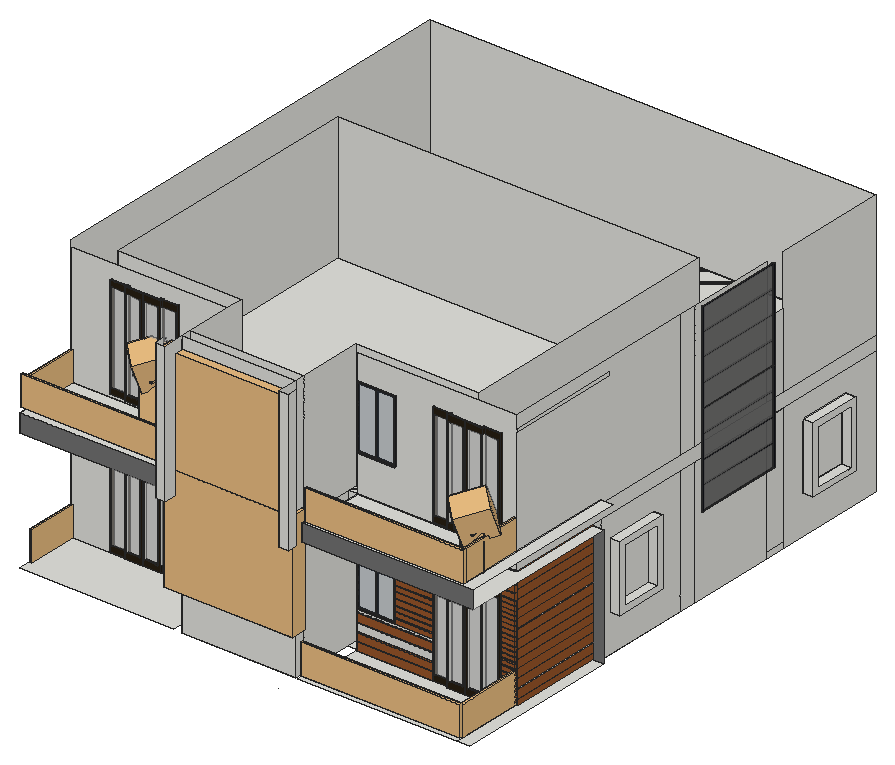
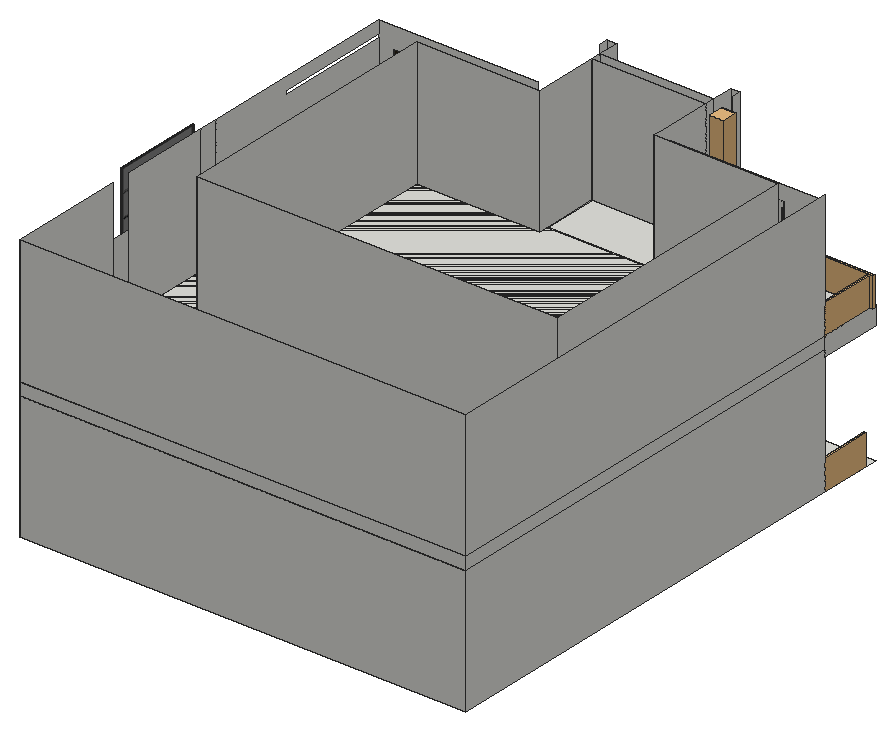
# SketchUp Ruby script. Lengths in inches.
U = 1.inch
M = Sketchup.active_model
def pt(a) = Geom::Point3d.new(a.map { |v| v * U })
def face(e, loops, mat)
  f = e.add_face(loops[0].map { |a| pt(a) })
  loops[1..].each { |l| e.add_face(l.map { |a| pt(a) }).erase! }
  f.material = f.back_material = mat if mat
  f
end
# faces: each face lists its corners as indices into pts; further lists are holes
def faces(e, pts, list, mat = nil) = list.each { |f| face(e, (f[0].is_a?(Array) ? f : [f]).map { |l| l.map { |i| pts[i] } }, mat) }
# xy, xz, yz: faces in a plane at the given z, y or x. An outline is a flat list of corners, or four numbers for a rectangle; further outlines are holes
def ring(l) = l.size == 4 ? [[l[0], l[1]], [l[2], l[1]], [l[2], l[3]], [l[0], l[3]]] : l.each_slice(2).to_a
def flat(e, list, mat, &to3) = list.each { |f| face(e, (f[0].is_a?(Array) ? f : [f]).map { |l| ring(l).map { |u, v| to3.(u, v) } }, mat) }
def xy(e, z, list, mat = nil) = flat(e, list, mat) { |x, y| [x, y, z] }
def xz(e, y, list, mat = nil) = flat(e, list, mat) { |x, z| [x, y, z] }
def yz(e, x, list, mat = nil) = flat(e, list, mat) { |y, z| [x, y, z] }
def lines(e, pts, list) = list.each { |a, b| e.add_line(pt(pts[a]), pt(pts[b])) }
# prism: a flat outline (further loops are holes) pulled along v
def prism(e, loops, v, mat = nil)
  f = face(e, loops, mat); d = Geom::Vector3d.new(v.map { |x| x * U })
  f.pushpull(f.normal.samedirection?(d) ? d.length : -d.length)
end
def box(e, o, s, mat = nil) = prism(e, [[o, [o[0] + s[0], o[1], o[2]], [o[0] + s[0], o[1] + s[1], o[2]], [o[0], o[1] + s[1], o[2]]]], [0, 0, s[2]], mat)
def at(x, y, z, deg = 0) = Geom::Transformation.translation(pt([x, y, z])) * Geom::Transformation.rotation(ORIGIN, Z_AXIS, deg.degrees)
def axes(o, x, y, z) = Geom::Transformation.new([*x, 0, *y, 0, *z, 0, *pt(o).to_a, 1])
def part(name) = M.definitions.add(name)
# library, detail: a bought-in or finely detailed component or shape, given as its bounding box
def library(name, o, s) = part(name).tap { |d| box(d.entities, o, s) }
def detail(e, o, s) = box(e.add_group.entities, o, s)
def put(e, d, t, mat = nil) = e.add_instance(d, t).tap { |i| i.material = mat if mat }
def group(e, t, mat = nil) = e.add_group.tap { |g| g.transformation = t; g.material = mat if mat }.entities
root = M.entities
M.materials.add("Material__1").color = [51, 42, 44]
M.materials.add("Material__2").color = [97, 132, 37]
M.materials.add("[0136_Charcoal]").color = [35, 35, 35]
M.materials.add("[Color M05]").color = [114, 114, 114]
M.materials.add("[Translucent Glass Gray]2").color = [201, 201, 201]
M.materials["[Translucent Glass Gray]2"].alpha = 0.5
M.materials.add("[Translucent_Glass_Blue]").color = [68, 104, 165]
M.materials["[Translucent_Glass_Blue]"].alpha = 0.07
M.materials.add("[Translucent_Glass_Green_Dark]").color = [33, 68, 103]
M.materials["[Translucent_Glass_Green_Dark]"].alpha = 0.08
M.materials.add("[Wood Cherry Original]").color = [152, 86, 42]
M.materials.add("oak swatch").color = [40, 31, 19]
M.materials.add("{045efeae-c101-a24d-bd9b-6f5600100adb}").color = [102, 102, 102]
M.materials["{045efeae-c101-a24d-bd9b-6f5600100adb}"].alpha = 0.7
M.materials.add("{16756a1b-d383-d94f-ad82-104813d2624f}").color = [19, 21, 27]
c1 = part("Group\#7")
box(c1.entities,[0,0,0],[1.77,4.72,80.31],"oak swatch")
c2 = part("Exterior Sliding Doors")
xy(c2.entities,0,[[1.77,33.07,3.54,70.87],[1.77,70.87,3.54,108.66]])
xy(c2.entities,0,[[0,0,1.77,33.07],[0,108.66,1.77,141.73]],"oak swatch")
xy(c2.entities,4.72,[[0,4.72,1.77,33.07],[1.77,37.8,3.54,66.14],[1.77,75.88,3.54,103.9375],[0,108.66,1.77,137.01]],"oak swatch")
xy(c2.entities,75.59,[[1.77,37.8,3.54,66.14],[1.77,75.88,3.54,103.9375]])
xy(c2.entities,75.59,[[0,4.72,1.77,33.07],[0,108.66,1.77,137.01]],"oak swatch")
xy(c2.entities,80.31,[[0,0,1.77,33.07],[1.77,33.07,3.54,70.87],[1.77,70.87,3.54,108.66],[0,108.66,1.77,141.73]],"oak swatch")
xz(c2.entities,0,[[0,0,1.77,80.31]],"oak swatch")
xz(c2.entities,4.72,[[0,4.72,1.77,75.59]],"oak swatch")
xz(c2.entities,33.07,[[0,0,1.77,4.72],[1.77,0,3.54,80.31],[0,75.59,1.77,80.31]],"oak swatch")
xz(c2.entities,37.8,[[1.77,4.72,3.54,75.59]])
xz(c2.entities,66.14,[[1.77,4.72,3.54,75.59]],"oak swatch")
xz(c2.entities,70.87,[[1.77,0,3.54,80.31]])
xz(c2.entities,75.88,[[1.77,4.72,3.54,75.59]])
xz(c2.entities,103.9375,[[1.77,4.72,3.54,75.59]],"oak swatch")
xz(c2.entities,108.66,[[1.77,4.72,3.54,75.59]])
xz(c2.entities,108.66,[[0,0,3.54,4.72],[0,75.59,3.54,80.31]],"oak swatch")
xz(c2.entities,137.01,[[0,4.72,1.77,75.59]],"oak swatch")
xz(c2.entities,141.73,[[0,0,1.77,80.31]],"oak swatch")
yz(c2.entities,0,[[0,0,33.07,0,33.07,4.72,4.72,4.72,4.72,75.59,33.07,75.59,33.07,80.31,0,80.31],[108.66,0,141.73,0,141.73,80.31,108.66,80.31,108.66,75.59,137.01,75.59,137.01,4.72,108.66,4.72]],"oak swatch")
yz(c2.entities,1.77,[[4.72,4.72,33.07,75.59],[37.8,4.72,66.14,75.59],[75.88,4.72,103.9375,75.59],[108.66,4.72,137.01,75.59]],"[Translucent Glass Gray]2")
yz(c2.entities,1.77,[[0,0,33.07,0,33.07,4.72,4.72,4.72,4.72,75.59,33.07,75.59,33.07,80.31,0,80.31],[[33.07,0,70.87,80.31],[37.8,4.72,66.14,75.59]],[[70.87,0,141.73,80.31],[108.66,4.72,137.01,75.59],[75.88,4.72,103.9375,75.59]]],"oak swatch")
yz(c2.entities,3.54,[[[33.07,0,70.87,80.31],[37.8,4.72,66.14,75.59]],[[70.87,0,108.66,80.31],[75.88,4.72,103.9375,75.59]]],"oak swatch")
put(c2.entities,c1,at(0,33.07,0))
put(c2.entities,c1,at(0,103.9375,0))
c3 = part("Group\#9")
box(c3.entities,[0,-1.5625,0],[72.51,1.5625,7.17])
c4 = library("Glass Railings(black Handrails)",[-57.04,-132.55,0],[169.29,2.52,28.17])
c5 = part("Group\#11")
box(c5.entities,[0,0,0],[14,3.63,1.625])
c6 = part("Group\#8")
box(c6.entities,[61.69,-1.625,-2],[88.94,1.625,7.49])
c7 = part("Group\#10")
box(c7.entities,[0,0,0],[36.2,4.62,1.5625])
c8 = part("Two-panel window \#1")
xy(c8.entities,-18,[[0,-31,2,35]],"[0136_Charcoal]")
xy(c8.entities,-16,[[0,-29,0.9375,33],[0.9375,-29,1.125,33],[1.125,-29,2,1],[1.125,3,2,33]],"[0136_Charcoal]")
xy(c8.entities,76,[[0,-29,0.9375,33],[0.9375,-29,1.125,33],[1.125,-29,2,1],[1.125,3,2,33]],"[0136_Charcoal]")
xy(c8.entities,78,[[0,-31,2,35]],"[0136_Charcoal]")
xz(c8.entities,-31,[[0,-18,2,78]],"[0136_Charcoal]")
xz(c8.entities,-29,[[0,-16,0.9375,76],[0.9375,-16,1.125,76],[1.125,-16,2,76]],"[0136_Charcoal]")
xz(c8.entities,1,[[1.125,-16,2,76]],"[0136_Charcoal]")
xz(c8.entities,3,[[1.125,-16,2,76]],"[0136_Charcoal]")
xz(c8.entities,33,[[0,-16,0.9375,76],[0.9375,-16,1.125,76],[1.125,-16,2,76]],"[0136_Charcoal]")
xz(c8.entities,35,[[0,-18,2,78]],"[0136_Charcoal]")
yz(c8.entities,0,[[[-31,-18,35,78],[-29,-16,33,76]]],"[0136_Charcoal]")
yz(c8.entities,0.9375,[[-29,-16,33,76]],"[Translucent_Glass_Blue]")
yz(c8.entities,1.125,[[1,-16,3,76]],"[0136_Charcoal]")
yz(c8.entities,1.125,[[-29,-16,1,76],[3,-16,33,76]],"[Translucent_Glass_Green_Dark]")
yz(c8.entities,2,[[[-31,-18,35,78],[-29,-16,1,76],[3,-16,33,76]]],"[0136_Charcoal]")
c9 = part("Two-panel window")
put(c9.entities,c8,axes([-31.84,50.72,0],[1,0,0],[0,1.1,0],[0,0,1]))
c10 = part("normal window")
put(c10.entities,c9,axes([114.26,44.3125,18],[0,1,0],[-0.90909,0,0],[0,0,1]))
c11 = part("Group\#20")
xy(c11.entities,0,[[[0,0,50.8125,62.9375],[5.49,5.49,45.32,57.45]],[5.49,5.49,45.32,57.45]])
xy(c11.entities,9.5625,[[[0,0,50.8125,62.9375],[5.49,5.49,45.32,57.45]]])
xz(c11.entities,0,[[0,0,50.8125,9.5625]])
xz(c11.entities,5.49,[[5.49,0,45.32,9.5625]])
xz(c11.entities,57.45,[[5.49,0,45.32,9.5625]])
xz(c11.entities,62.9375,[[0,0,50.8125,9.5625]])
yz(c11.entities,0,[[0,0,62.9375,9.5625]])
yz(c11.entities,5.49,[[5.49,0,57.45,9.5625]])
yz(c11.entities,45.32,[[5.49,0,57.45,9.5625]])
yz(c11.entities,50.8125,[[0,0,62.9375,9.5625]])
c12 = library("Facade Louver",[-2.17,-1,-2.17],[122.45,14.39,102.76])
c13 = part("Furniture_0DcpanrIvuI8n_9Ae92L5A")
g1 = group(c13.entities,at(0,0,0))
box(g1,[-19.29,-0.2,0.39],[38.58,0.4,83.86],"{045efeae-c101-a24d-bd9b-6f5600100adb}")
g2 = group(c13.entities,at(0,0,0))
box(g2,[-19.68,-0.59,63.39],[39.36,1.18,0.39],"{16756a1b-d383-d94f-ad82-104813d2624f}")
box(g2,[-19.68,-0.59,42.52],[39.36,1.18,0.39],"{16756a1b-d383-d94f-ad82-104813d2624f}")
box(g2,[-19.68,-0.59,21.26],[39.36,1.18,0.39],"{16756a1b-d383-d94f-ad82-104813d2624f}")
xy(g2,0,[[-19.68,-0.59,19.68,0.59]],"{16756a1b-d383-d94f-ad82-104813d2624f}")
xy(g2,0.39,[[-19.68,-0.59,-19.29,0.59],[-19.68,-0.59,19.68,0.59],[19.29,-0.59,19.68,0.59]],"{16756a1b-d383-d94f-ad82-104813d2624f}")
xy(g2,84.25,[[-19.68,-0.59,19.68,0.59]],"{16756a1b-d383-d94f-ad82-104813d2624f}")
xy(g2,84.65,[[-19.68,-0.59,-19.29,0.59],[-19.68,-0.59,19.68,0.59],[19.29,-0.59,19.68,0.59]],"{16756a1b-d383-d94f-ad82-104813d2624f}")
xz(g2,-0.59,[[-19.68,0,19.68,0.39],[-19.68,0.39,-19.29,84.65],[19.29,0.39,19.68,84.65],[-19.68,84.25,19.68,84.65]],"{16756a1b-d383-d94f-ad82-104813d2624f}")
xz(g2,0.59,[[-19.68,0,19.68,0.39],[-19.68,0.39,-19.29,84.65],[19.29,0.39,19.68,84.65],[-19.68,84.25,19.68,84.65]],"{16756a1b-d383-d94f-ad82-104813d2624f}")
yz(g2,-19.68,[[-0.59,0,0.59,0.39],[-0.59,0.39,0.59,84.65],[-0.59,84.25,0.59,84.65]],"{16756a1b-d383-d94f-ad82-104813d2624f}")
yz(g2,-19.29,[[-0.59,0.39,0.59,84.65]],"{16756a1b-d383-d94f-ad82-104813d2624f}")
yz(g2,19.29,[[-0.59,0.39,0.59,84.65]],"{16756a1b-d383-d94f-ad82-104813d2624f}")
yz(g2,19.68,[[-0.59,0,0.59,0.39],[-0.59,0.39,0.59,84.65],[-0.59,84.25,0.59,84.65]],"{16756a1b-d383-d94f-ad82-104813d2624f}")
c14 = part("Glass Window")
put(c14.entities,c13,at(0,0,-42.32))
c15 = part("Group\#19")
box(c15.entities,[0,-1.625,0],[150.625,1.625,5.49])
c16 = library("\#1",[-138.85,-135.75,0],[277.7,270.97,9.64])
c17 = library("\#2",[-34.84,-73.35,-33.91],[69.68,146.26,68.31])
c18 = library("\#5",[-4127.85,-1300.75,-2324.72],[5349.84,4521.24,5423.31])
c19 = part("\#3")
put(c19.entities,c18,at(450.18,-1111.4375,0),"Material__2")
c20 = part("12")
put(c20.entities,c16,axes([-49.79,-36.9375,349.64],[0.59279,0,0],[0,0.59279,0],[0,0,0.59279]),"Material__1")
put(c20.entities,c17,axes([-39.24,-18.18,177.19],[1.20819,-2.09264,0],[0,0,2.41638],[2.09264,1.20819,0]))
put(c20.entities,c19,axes([-83.44,-46.04,442.44],[-0.03636,-0.03293,-0.01473],[-0.00083,-0.02391,0.05549],[0.02997,-0.02791,-0.01158]))
xy(root,132,[[200.76,112.2,308.76,121.2],[45.88,113.44,191.76,173.57],[317.76,113.44,468.38,173.57],[200.76,121.2,308.76,121.2,308.76,182.57,425.76,182.57,425.76,442.69,83.76,442.69,83.76,182.57,200.76,182.57],[191.76,151.89,200.76,151.89,200.76,182.57,83.76,182.57,83.76,442.69,425.76,442.69,425.76,182.57,308.76,182.57,308.76,173.57,468.38,173.57,468.38,598.82,45.88,598.82,45.88,173.57,191.76,173.57]])
xy(root,138.375,[[317.76,103.01,468.38,113.44],[468.38,103.01,480.01,261.76]])
xy(root,246.8125,[[45.88,113.44,191.76,173.57]])
xy(root,252,[[317.76,107.51,317.76,173.57,468.38,173.57,468.38,261.76,480.01,261.76,480.01,107.51],[200.76,112.2,308.76,121.2],[45.88,173.57,200.76,173.57,200.76,182.57,83.76,182.57,83.76,442.69,425.76,442.69,425.76,182.57,308.76,182.57,308.76,173.57,468.38,173.57,468.38,598.82,45.88,598.82]])
xy(root,264,[[200.76,112.2,308.76,121.2],[45.88,113.44,191.76,173.57],[317.76,113.44,468.38,173.57],[200.76,121.2,308.76,121.2,308.76,182.57,425.76,182.57,425.76,442.69,83.76,442.69,83.76,182.57,200.76,182.57],[45.88,173.57,200.76,173.57,200.76,182.57,83.76,182.57,83.76,442.69,425.76,442.69,425.76,182.57,308.76,182.57,308.76,173.57,468.38,173.57,468.38,598.82,45.88,598.82]])
xy(root,268.25,[[317.76,107.51,480.01,107.51,480.01,273.38,468.38,273.38,468.38,113.44,317.76,113.44]])
xz(root,91.69,[[191.76,252,200.76,383.9375],[308.76,252,317.76,384]])
xz(root,107.51,[[317.76,252,480.01,268.25]],"[Color M05]")
xz(root,112.2,[[200.76,132,308.76,252],[200.76,252,308.76,264],[200.76,264,308.76,384]])
xz(root,113.44,[[317.76,132,468.38,138.375],[317.76,264,468.38,268.25]])
xz(root,113.44,[[45.88,246.8125,191.76,264]],"[Color M05]")
xz(root,121.2,[[200.76,132,308.76,252],[200.76,264,308.76,384]])
xz(root,173.57,[[45.88,132,191.76,246.8125],[390.27,132,468.38,132,468.38,246.51,317.76,246.51,317.76,139.17,390.27,139.17],[45.88,246.8125,191.76,252],[191.76,252,200.76,264],[308.76,252,317.76,264],
  [317.76,252,468.38,264],[45.88,264,191.76,378.5],[317.76,264,468.38,384]])
xz(root,182.57,[[83.76,132,200.76,252],[308.76,132,425.76,252],[83.76,264,200.76,384],[308.76,264,425.76,384]])
xz(root,261.76,[[468.38,138.375,480.01,252]],"[Color M05]")
xz(root,442.69,[[83.76,132,425.76,252],[83.76,264,425.76,384]])
xz(root,598.82,[[45.88,132,468.38,252],[45.88,264,468.38,384]])
yz(root,45.88,[[173.57,132,598.82,252],[113.44,246.8125,173.57,264],[173.57,264,598.82,384]])
yz(root,83.76,[[182.57,132,442.69,252],[182.57,264,442.69,384]])
yz(root,191.76,[[113.44,246.8125,173.57,264],[91.69,252,100.69,383.9375]])
yz(root,200.76,[[112.2,132,121.2,252],[121.2,132,182.57,252],[91.69,252,112.2,383.9375],[112.2,252,121.2,264],[121.2,252,173.57,264],
  [112.2,264,121.2,383.9375],[121.2,264,182.57,264,182.57,384,173.57,384,173.57,383.9375,121.2,383.9375]])
yz(root,308.76,[[112.2,132,121.2,252],[121.2,132,182.57,252],[91.69,252,112.2,384],[112.2,252,121.2,264],[121.2,252,173.57,264],
  [112.2,264,121.2,384],[121.2,264,182.57,384]])
yz(root,317.76,[[91.69,252,100.69,252,100.69,369.07,100.51,369.07,100.51,372.57,100.69,372.57,100.69,384,91.69,384],[107.51,252,173.57,252,173.57,264,113.44,264,113.44,268.25,107.51,268.25]])
yz(root,425.76,[[182.57,132,442.69,252],[182.57,264,442.69,384]])
yz(root,468.38,[[113.44,132,173.57,138.375],[173.57,132,261.76,138.375],[261.76,132,273.38,252],[273.38,132,367.14,252],[367.14,132,384.58,252],
  [384.58,132,469.33,252],[469.33,132,488.7,138.25],[488.7,132,598.82,252],[469.33,138.25,488.7,250.375],[173.57,138.375,261.76,252],
  [469.33,250.375,488.7,252],[173.57,252,273.38,264],[367.14,252,384.58,264],[469.33,252,488.7,264],[113.44,264,173.57,268.25],
  [173.57,264,273.38,268.25],[273.38,264,367.14,264,367.14,384,173.57,384,173.57,372.57,283.99,372.57,283.99,369.07,173.57,369.07,173.57,268.25,273.38,268.25],[367.14,264,384.58,384],[384.58,264,469.33,384],[469.33,264,488.7,335.6875],
  [488.7,264,598.82,384]])
p = [[308.59,91.69,131.75],[308.59,91.69,132]]
lines(root,p,[[0,1]])
put(root,c2,axes([390.27,173.57,132],[0,-1,0],[0.4524,0,0],[0,0,1.21]))
put(root,c3,at(317.76,173.57,132),"[Wood Cherry Original]")
put(root,c4,axes([-84.15,141.22,132.11],[0,0.28822,0],[-1,0,0],[0,0,1]))
put(root,c5,axes([454.38,173.57,132.2],[1,0,0],[0,0,1],[0,-1,0]),"[Wood Cherry Original]")
put(root,c2,axes([84.67,173.57,133.875],[0,-1,0],[0.4524,0,0],[0,0,1.21]))
put(root,c6,at(467.95,111.88,136.88,90),"[Wood Cherry Original]")
put(root,c4,axes([335.83,130.93,138.375],[0,0.37992,0],[-1,0,0],[0,0,1]))
put(root,c4,axes([368.27,239.28,139.26],[0.89,0,0],[0,1,0],[0,0,1]))
put(root,c3,at(317.76,173.57,140.0625),"[Wood Cherry Original]")
put(root,c5,axes([454.38,173.57,140.26],[1,0,0],[0,0,1],[0,-1,0]),"[Wood Cherry Original]")
put(root,c6,at(467.95,111.88,145.69,90),"[Wood Cherry Original]")
put(root,c5,axes([454.38,173.57,145.07],[1,0,0],[0,0,1],[0,-1,0]),"[Wood Cherry Original]")
put(root,c3,at(317.76,173.57,148.4375),"[Wood Cherry Original]")
put(root,c3,at(317.82,173.57,148.4375))
put(root,c5,axes([454.38,173.57,149.63],[1,0,0],[0,0,1],[0,-1,0]),"[Wood Cherry Original]")
put(root,c6,at(467.95,111.88,154.69,90),"[Wood Cherry Original]")
put(root,c5,axes([454.38,173.57,154.13],[1,0,0],[0,0,1],[0,-1,0]),"[Wood Cherry Original]")
put(root,c3,at(317.76,173.57,156.5625),"[Wood Cherry Original]")
put(root,c5,axes([454.38,173.57,158.82],[1,0,0],[0,0,1],[0,-1,0]),"[Wood Cherry Original]")
put(root,c6,at(467.95,111.88,163.13,90),"[Wood Cherry Original]")
put(root,c5,axes([454.38,173.57,163.76],[1,0,0],[0,0,1],[0,-1,0]),"[Wood Cherry Original]")
put(root,c7,axes([354.07,173.57,167.03],[1,0,0],[0,0,1],[0,-1,0]),"[Wood Cherry Original]")
put(root,c10,axes([299.72,167.1875,167.03],[0.5481,0,0],[0,0.441,0],[0,0,0.63]))
put(root,c11,axes([468.38,283.99,168.58],[0,1,0],[0,0,1],[1,0,0]))
put(root,c11,axes([468.38,512.67,168.58],[0,1,0],[0,0,1],[1,0,0]))
put(root,c6,at(467.95,111.88,171.26,90),"[Wood Cherry Original]")
put(root,c5,axes([454.38,173.57,169.38],[1,0,0],[0,0,1],[0,-1,0]),"[Wood Cherry Original]")
put(root,c12,at(192.27,104.35,173.41))
put(root,c7,axes([354.06,173.57,173.17],[1,0,0],[0,0,1],[0,-1,0]),"[Wood Cherry Original]")
put(root,c5,axes([454.38,173.57,175.33],[1,0,0],[0,0,1],[0,-1,0]),"[Wood Cherry Original]")
put(root,c6,at(467.95,111.88,179.38,90),"[Wood Cherry Original]")
put(root,c7,axes([354.41,173.57,178.4],[1,0,0],[0,0,1],[0,-1,0]),"[Wood Cherry Original]")
put(root,c5,axes([454.38,173.57,179.52],[1,0,0],[0,0,1],[0,-1,0]),"[Wood Cherry Original]")
put(root,c7,axes([354.07,173.57,183.5625],[1,0,0],[0,0,1],[0,-1,0]),"[Wood Cherry Original]")
put(root,c5,axes([454.38,173.57,183.83],[1,0,0],[0,0,1],[0,-1,0]),"[Wood Cherry Original]")
put(root,c6,at(467.95,111.88,188.07,90),"[Wood Cherry Original]")
put(root,c5,axes([454.38,173.57,188.14],[1,0,0],[0,0,1],[0,-1,0]),"[Wood Cherry Original]")
put(root,c7,axes([354.07,173.57,189.5625],[1,0,0],[0,0,1],[0,-1,0]),"[Wood Cherry Original]")
put(root,c5,axes([454.38,173.57,192.27],[1,0,0],[0,0,1],[0,-1,0]),"[Wood Cherry Original]")
put(root,c6,at(467.95,111.88,196.76,90),"[Wood Cherry Original]")
put(root,c7,axes([354.07,173.57,195],[1,0,0],[0,0,1],[0,-1,0]),"[Wood Cherry Original]")
put(root,c5,axes([454.38,173.57,196.58],[1,0,0],[0,0,1],[0,-1,0]),"[Wood Cherry Original]")
put(root,c7,axes([354.07,173.57,200.75],[1,0,0],[0,0,1],[0,-1,0]),"[Wood Cherry Original]")
put(root,c5,axes([454.38,173.57,201.02],[1,0,0],[0,0,1],[0,-1,0]),"[Wood Cherry Original]")
put(root,c6,at(467.95,111.88,205.51,90),"[Wood Cherry Original]")
put(root,c5,axes([454.38,173.57,205.45],[1,0,0],[0,0,1],[0,-1,0]),"[Wood Cherry Original]")
put(root,c7,axes([354.07,171.8,206.73],[1,0,0],[0,0,1],[0,-1,0]),"[Wood Cherry Original]")
put(root,c5,axes([454.38,173.57,209.77],[1,0,0],[0,0,1],[0,-1,0]),"[Wood Cherry Original]")
put(root,c14,axes([475.3125,426.95,255.15],[0,-2.15265,0],[1,0,0],[0,0,1.03]))
put(root,c6,at(467.95,111.88,213.7,90),"[Wood Cherry Original]")
put(root,c7,axes([354.07,171.8,212.05],[1,0,0],[0,0,1],[0,-1,0]),"[Wood Cherry Original]")
put(root,c5,axes([454.38,173.57,214.02],[1,0,0],[0,0,1],[0,-1,0]),"[Wood Cherry Original]")
put(root,c7,axes([354.07,173.57,216.88],[1,0,0],[0,0,1],[0,-1,0]),"[Wood Cherry Original]")
put(root,c5,axes([454.38,173.57,218.14],[1,0,0],[0,0,1],[0,-1,0]),"[Wood Cherry Original]")
put(root,c6,at(467.95,111.88,222.14,90),"[Wood Cherry Original]")
put(root,c7,axes([354.07,171.8,222.46],[1,0,0],[0,0,1],[0,-1,0]),"[Wood Cherry Original]")
put(root,c5,axes([454.38,173.57,222.52],[1,0,0],[0,0,1],[0,-1,0]),"[Wood Cherry Original]")
put(root,c15,at(317.76,173.57,227.39),"[Wood Cherry Original]")
put(root,c6,at(467.95,111.88,230.33,90),"[Wood Cherry Original]")
put(root,c15,at(317.76,173.57,233.83),"[Wood Cherry Original]")
put(root,c6,at(467.95,111.88,238.51,90),"[Wood Cherry Original]")
put(root,c15,at(317.76,173.57,240.27),"[Wood Cherry Original]")
put(root,c6,at(467.95,111.88,246.51,90),"[Wood Cherry Original]")
put(root,c15,at(317.76,173.57,246.51),"[Wood Cherry Original]")
g3 = group(root,at(74.76,451.69,252))
box(g3,[-28.875,-278.125,0],[422.5,425.25,12])
put(root,c20,axes([459.03,141.87,260.3],[0.1092,0,0],[0,0.1092,0],[0,0,0.1092]))
put(root,c20,axes([132.26,170.44,262.67],[0.1092,0,0],[0,0.1092,0],[0,0,0.1092]))
put(root,c4,axes([-84.15,138.77,263.79],[0,0.31005,0],[-1,0,0],[0,0,1]))
put(root,c4,axes([93.65,251.23,265.25],[0.89,0,0],[0,1,0],[0,0,1]))
put(root,c2,axes([390.27,173.57,266.75],[0,-1,0],[0.4524,0,0],[0,0,1.21]))
put(root,c2,axes([84.67,173.57,267.625],[0,-1,0],[0.4524,0,0],[0,0,1.21]))
put(root,c4,axes([368.53,243.48,268.25],[0.89,0,0],[0,1,0],[0,0,1]))
put(root,c4,axes([335.83,132.73,268.25],[0,0.36382,0],[-1,0,0],[0,0,1]))
put(root,c12,at(188.27,104.35,272.47))
put(root,c14,axes([475.3125,426.95,341.93],[0,-2.15265,0],[1,0,0],[0,0,1.03]))
put(root,c10,axes([299.72,167.1875,299.6],[0.5481,0,0],[0,0.441,0],[0,0,0.63]))
